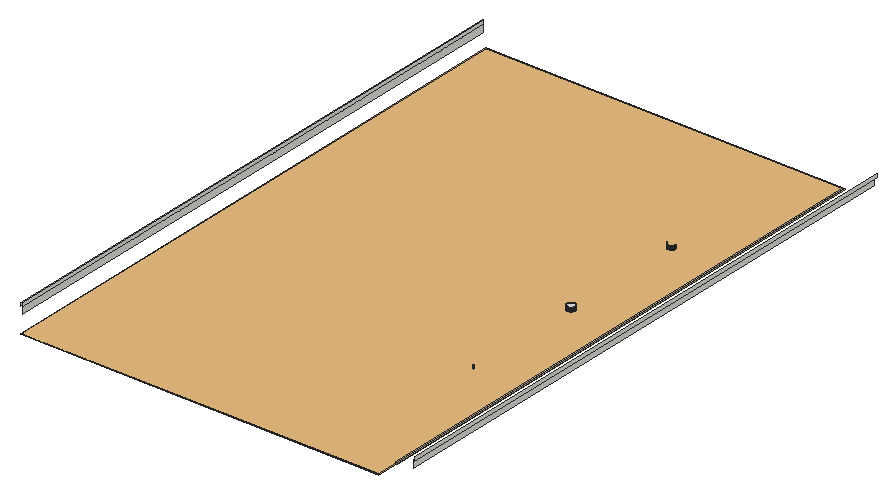
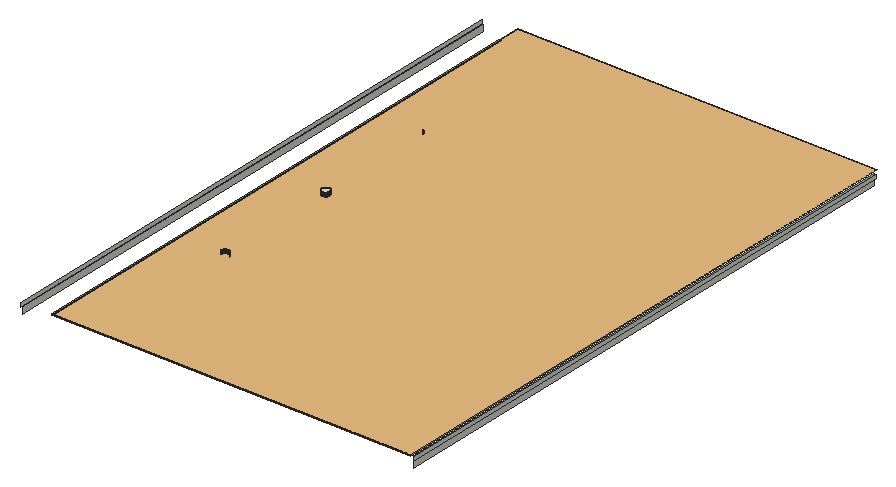
# SketchUp Ruby script. Lengths in inches.
U = 1.inch
M = Sketchup.active_model
def pt(a) = Geom::Point3d.new(a.map { |v| v * U })
def face(e, loops, mat)
  f = e.add_face(loops[0].map { |a| pt(a) })
  loops[1..].each { |l| e.add_face(l.map { |a| pt(a) }).erase! }
  f.material = f.back_material = mat if mat
  f
end
# faces: each face lists its corners as indices into pts; further lists are holes
def faces(e, pts, list, mat = nil) = list.each { |f| face(e, (f[0].is_a?(Array) ? f : [f]).map { |l| l.map { |i| pts[i] } }, mat) }
# xy, xz, yz: faces in a plane at the given z, y or x. An outline is a flat list of corners, or four numbers for a rectangle; further outlines are holes
def ring(l) = l.size == 4 ? [[l[0], l[1]], [l[2], l[1]], [l[2], l[3]], [l[0], l[3]]] : l.each_slice(2).to_a
def flat(e, list, mat, &to3) = list.each { |f| face(e, (f[0].is_a?(Array) ? f : [f]).map { |l| ring(l).map { |u, v| to3.(u, v) } }, mat) }
def xy(e, z, list, mat = nil) = flat(e, list, mat) { |x, y| [x, y, z] }
def xz(e, y, list, mat = nil) = flat(e, list, mat) { |x, z| [x, y, z] }
def yz(e, x, list, mat = nil) = flat(e, list, mat) { |y, z| [x, y, z] }
def lines(e, pts, list) = list.each { |a, b| e.add_line(pt(pts[a]), pt(pts[b])) }
# prism: a flat outline (further loops are holes) pulled along v
def prism(e, loops, v, mat = nil)
  f = face(e, loops, mat); d = Geom::Vector3d.new(v.map { |x| x * U })
  f.pushpull(f.normal.samedirection?(d) ? d.length : -d.length)
end
def box(e, o, s, mat = nil) = prism(e, [[o, [o[0] + s[0], o[1], o[2]], [o[0] + s[0], o[1] + s[1], o[2]], [o[0], o[1] + s[1], o[2]]]], [0, 0, s[2]], mat)
def at(x, y, z, deg = 0) = Geom::Transformation.translation(pt([x, y, z])) * Geom::Transformation.rotation(ORIGIN, Z_AXIS, deg.degrees)
def axes(o, x, y, z) = Geom::Transformation.new([*x, 0, *y, 0, *z, 0, *pt(o).to_a, 1])
def part(name) = M.definitions.add(name)
# library, detail: a bought-in or finely detailed component or shape, given as its bounding box
def library(name, o, s) = part(name).tap { |d| box(d.entities, o, s) }
def detail(e, o, s) = box(e.add_group.entities, o, s)
def put(e, d, t, mat = nil) = e.add_instance(d, t).tap { |i| i.material = mat if mat }
def group(e, t, mat = nil) = e.add_group.tap { |g| g.transformation = t; g.material = mat if mat }.entities
root = M.entities
M.materials.add("False ceiling Light").color = [253, 207, 127]
c1 = library("Group\#41",[0,0,-0.5],[265,430,0.5])
xy(root,351,[[251.84,435,251.76,435.01,251.6875,435.02,251.61,435.03,251.45,435.05,251.375,435.07,251.3,435.08,251.22,435.1,251.15,435.125,251.07,435.15,251,435.17,250.92,435.2,250.71,435.29,250.64,435.33,250.57,435.36,250.43,435.44,250.37,435.48,250.3,435.53,250.24,435.57,250.17,435.62,249.93,435.82,249.88,435.88,249.77,435.99,249.62,436.17,249.57,436.24,249.53,436.3,249.48,436.37,249.44,436.43,249.36,436.57,249.33,436.64,249.29,436.71,249.23,436.85,249.2,436.93,249.17,437,249.15,437.07,249.125,437.15,249.1,437.22,249.08,437.3,249.07,437.375,249.05,437.45,249.03,437.61,249.02,437.6875,249.01,437.76,249,437.84,249,438.16,249.01,438.24,249.02,438.3125,249.03,438.39,249.05,438.55,249.07,438.625,249.08,438.7,249.1,438.78,249.125,438.85,249.15,438.93,249.17,439,249.2,439.08,249.29,439.29,249.33,439.36,249.36,439.43,249.44,439.57,249.48,439.63,249.53,439.7,249.57,439.76,249.62,439.83,249.82,440.07,249.88,440.12,249.99,440.23,250.17,440.38,250.24,440.43,250.3,440.47,250.37,440.52,250.43,440.56,250.57,440.64,250.64,440.67,250.71,440.71,250.85,440.77,250.93,440.8,251,440.83,251.07,440.85,251.15,440.875,251.22,440.9,251.3,440.92,251.375,440.93,251.45,440.95,251.61,440.97,251.6875,440.98,251.76,440.99,251.84,441,252.16,441,252.24,440.99,252.3125,440.98,252.39,440.97,252.55,440.95,252.625,440.93,252.7,440.92,252.78,440.9,252.85,440.875,252.93,440.85,253,440.83,253.08,440.8,253.29,440.71,253.36,440.67,253.43,440.64,253.57,440.56,253.63,440.52,253.7,440.47,253.76,440.43,253.83,440.38,254.07,440.18,254.12,440.12,254.23,440.01,254.38,439.83,254.43,439.76,254.47,439.7,254.52,439.63,254.56,439.57,254.64,439.43,254.67,439.36,254.71,439.29,254.77,439.15,254.8,439.07,254.83,439,254.85,438.93,254.875,438.85,254.9,438.78,254.92,438.7,254.93,438.625,254.95,438.55,254.97,438.39,254.98,438.3125,254.99,438.24,255,438.16,255,437.84,254.99,437.76,254.98,437.6875,254.97,437.61,254.95,437.45,254.93,437.375,254.92,437.3,254.9,437.22,254.875,437.15,254.85,437.07,254.83,437,254.8,436.92,254.71,436.71,254.67,436.64,254.64,436.57,254.56,436.43,254.52,436.37,254.47,436.3,254.43,436.24,254.38,436.17,254.18,435.93,254.12,435.88,254.01,435.77,253.83,435.62,253.76,435.57,253.7,435.53,253.63,435.48,253.57,435.44,253.43,435.36,253.36,435.33,253.29,435.29,253.15,435.23,253.07,435.2,253,435.17,252.93,435.15,252.85,435.125,252.78,435.1,252.7,435.08,252.625,435.07,252.55,435.05,252.39,435.03,252.3125,435.02,252.24,435.01,252.16,435]])
xz(root,348,[[251.84,348,251.92,351],[251.92,348,252,351],[252,348,252.08,351],[252.08,348,252.16,351]])
xz(root,435,[[251.84,348,251.92,351],[251.92,348,252,351],[252,348,252.08,351],[252.08,348,252.16,351]])
xz(root,441,[[251.84,348,251.92,351],[251.92,348,252,351],[252,348,252.08,351],[252.08,348,252.16,351]])
xz(root,528,[[251.84,348,251.92,351],[251.92,348,252,351],[252,348,252.08,351],[252.08,348,252.16,351]])
yz(root,9,[[234,354.5,660,357]])
yz(root,10,[[234,349.5,659,354.5],[234,354.5,659,357]])
yz(root,249,[[437.84,348,437.92,351],[437.92,348,438,351],[438,348,438.08,351],[438.08,348,438.16,351]])
yz(root,255,[[437.84,348,437.92,351],[437.92,348,438,351],[438,348,438.08,351],[438.08,348,438.16,351]])
yz(root,286,[[234,348,646,348.5]])
yz(root,287,[[234,348,647,348.5]])
yz(root,299,[[234,349.5,659,354.5]])
yz(root,300,[[234,354.5,660,357]])
p = [[251.45,347.95,348],[251.53,347.96,348],[251.53,347.96,351],[251.45,347.95,351],[251.61,347.97,348],[251.61,347.97,351],
  [251.6875,347.98,348],[251.6875,347.98,351],[251.76,347.99,348],[251.76,347.99,351],[251.84,348,348],[251.84,348,351],
  [252.24,347.99,348],[252.3125,347.98,348],[252.3125,347.98,351],[252.24,347.99,351],[252.16,348,348],[252.16,348,351],
  [252.39,347.97,348],[252.39,347.97,351],[252.47,347.96,348],[252.47,347.96,351],[251.61,435.03,348],[251.53,435.04,348],
  [251.53,435.04,351],[251.61,435.03,351],[251.45,435.05,348],[251.45,435.05,351],[251.6875,435.02,348],[251.6875,435.02,351],
  [251.76,435.01,348],[251.76,435.01,351],[251.84,435,348],[251.84,435,351],[252.24,435.01,348],[252.16,435,348],
  [252.16,435,351],[252.24,435.01,351],[252.3125,435.02,348],[252.3125,435.02,351],[252.39,435.03,348],[252.39,435.03,351],
  [252.47,435.04,348],[252.47,435.04,351],[252.55,435.05,348],[252.55,435.05,351],[251.07,435.15,348],[251,435.17,348],
  [251,435.17,351],[251.07,435.15,351],[251.22,435.1,348],[251.15,435.125,348],[251.15,435.125,351],[251.22,435.1,351],
  [251.3,435.08,348],[251.3,435.08,351],[251.375,435.07,348],[251.375,435.07,351],[252.625,435.07,348],[252.625,435.07,351],
  [252.7,435.08,348],[252.7,435.08,351],[252.78,435.1,348],[252.78,435.1,351],[252.85,435.125,348],[252.85,435.125,351],
  [252.93,435.15,348],[252.93,435.15,351],[253,435.17,348],[253,435.17,351],[250.85,435.23,348],[250.78,435.26,348],
  [250.78,435.26,351],[250.85,435.23,351],[250.92,435.2,348],[250.92,435.2,351],[253.07,435.2,348],[253.07,435.2,351],
  [253.15,435.23,348],[253.15,435.23,351],[253.22,435.26,348],[253.22,435.26,351],[250.71,435.29,348],[250.64,435.33,348],
  [250.64,435.33,351],[250.71,435.29,351],[250.57,435.36,348],[250.57,435.36,351],[253.29,435.29,348],[253.29,435.29,351],
  [253.36,435.33,348],[253.36,435.33,351],[253.43,435.36,348],[253.43,435.36,351],[250.5,435.4,348],[250.43,435.44,348],
  [250.43,435.44,351],[250.5,435.4,351],[250.37,435.48,348],[250.37,435.48,351],[253.5,435.4,348],[253.5,435.4,351],
  [253.57,435.44,348],[253.57,435.44,351],[253.63,435.48,348],[253.63,435.48,351],[250.3,435.53,348],[250.24,435.57,348],
  [250.24,435.57,351],[250.3,435.53,351],[253.7,435.53,348],[253.7,435.53,351],[253.76,435.57,348],[253.76,435.57,351],
  [250.17,435.62,348],[250.11,435.67,348],[250.11,435.67,351],[250.17,435.62,351],[253.83,435.62,348],[253.83,435.62,351],
  [253.89,435.67,348],[253.89,435.67,351],[250.05,435.72,348],[249.99,435.77,348],[249.99,435.77,351],[250.05,435.72,351],
  [253.95,435.72,348],[253.95,435.72,351],[254.01,435.77,348],[254.01,435.77,351],[249.93,435.82,348],[249.93,435.82,351],
  [249.88,435.88,348],[249.88,435.88,351],[254.06,435.82,348],[254.06,435.82,351],[254.12,435.88,348],[254.12,435.88,351],
  [249.82,435.94,348],[249.82,435.94,351],[249.77,435.99,348],[249.77,435.99,351],[254.18,435.93,348],[254.18,435.93,351],
  [254.23,435.99,348],[254.23,435.99,351],[249.72,436.05,348],[249.72,436.05,351],[254.28,436.05,348],[254.28,436.05,351],
  [249.67,436.11,348],[249.62,436.17,348],[249.62,436.17,351],[249.67,436.11,351],[254.33,436.11,348],[254.33,436.11,351],
  [254.38,436.17,348],[254.38,436.17,351],[249.57,436.24,348],[249.53,436.3,348],[249.53,436.3,351],[249.57,436.24,351],
  [254.43,436.24,348],[254.43,436.24,351],[254.47,436.3,348],[254.47,436.3,351],[249.48,436.37,348],[249.48,436.37,351],
  [254.52,436.37,348],[254.52,436.37,351],[249.44,436.43,348],[249.44,436.43,351],[249.4,436.5,348],[249.4,436.5,351],
  [254.56,436.43,348],[254.56,436.43,351],[254.6,436.5,348],[254.6,436.5,351],[249.36,436.57,348],[249.36,436.57,351],
  [254.64,436.57,348],[254.64,436.57,351],[249.33,436.64,348],[249.33,436.64,351],[249.29,436.71,348],[249.29,436.71,351],
  [254.67,436.64,348],[254.67,436.64,351],[254.71,436.71,348],[254.71,436.71,351],[249.26,436.78,348],[249.26,436.78,351],
  [254.74,436.78,348],[254.74,436.78,351],[249.23,436.85,348],[249.23,436.85,351],[254.77,436.85,348],[254.77,436.85,351],
  [249.2,436.93,348],[249.2,436.93,351],[249.17,437,348],[249.17,437,351],[254.8,436.92,348],[254.8,436.92,351],
  [254.83,437,348],[254.83,437,351],[249.15,437.07,348],[249.15,437.07,351],[254.85,437.07,348],[254.85,437.07,351],
  [249.125,437.15,348],[249.125,437.15,351],[249.1,437.22,348],[249.1,437.22,351],[254.875,437.15,348],[254.875,437.15,351],
  [254.9,437.22,348],[254.9,437.22,351],[249.08,437.3,348],[249.08,437.3,351],[254.92,437.3,348],[254.92,437.3,351],
  [249.07,437.375,348],[249.07,437.375,351],[254.93,437.375,348],[254.93,437.375,351],[249.05,437.45,348],[249.05,437.45,351],
  [254.95,437.45,348],[254.95,437.45,351],[249.04,437.53,348],[249.04,437.53,351],[249.03,437.61,348],[249.03,437.61,351],
  [254.96,437.53,348],[254.96,437.53,351],[254.97,437.61,348],[254.97,437.61,351],[249.02,437.6875,348],[249.02,437.6875,351],
  [254.98,437.6875,348],[254.98,437.6875,351],[249.01,437.76,348],[249.01,437.76,351],[254.99,437.76,348],[254.99,437.76,351],
  [249,437.84,348],[249,437.84,351],[255,437.84,348],[255,437.84,351],[249,438.16,348],[249.01,438.24,348],
  [249.01,438.24,351],[249,438.16,351],[249.02,438.3125,348],[249.02,438.3125,351],[254.99,438.24,348],[255,438.16,348],
  [255,438.16,351],[254.99,438.24,351],[254.98,438.3125,348],[254.98,438.3125,351],[249.03,438.39,348],[249.03,438.39,351],
  [254.97,438.39,348],[254.97,438.39,351],[249.04,438.47,348],[249.04,438.47,351],[254.96,438.47,348],[254.96,438.47,351],
  [249.05,438.55,348],[249.05,438.55,351],[249.07,438.625,348],[249.07,438.625,351],[254.95,438.55,348],[254.95,438.55,351],
  [254.93,438.625,348],[254.93,438.625,351],[249.08,438.7,348],[249.08,438.7,351],[254.92,438.7,348],[254.92,438.7,351],
  [249.1,438.78,348],[249.1,438.78,351],[254.9,438.78,348],[254.9,438.78,351],[249.125,438.85,348],[249.125,438.85,351],
  [254.875,438.85,348],[254.875,438.85,351],[249.15,438.93,348],[249.15,438.93,351],[249.17,439,348],[249.17,439,351],
  [254.83,439,348],[254.85,438.93,348],[254.85,438.93,351],[254.83,439,351],[249.2,439.08,348],[249.2,439.08,351],
  [254.8,439.07,348],[254.8,439.07,351],[249.23,439.15,348],[249.23,439.15,351],[249.26,439.22,348],[249.26,439.22,351],
  [254.74,439.22,348],[254.77,439.15,348],[254.77,439.15,351],[254.74,439.22,351],[249.29,439.29,348],[249.29,439.29,351],
  [254.71,439.29,348],[254.71,439.29,351],[249.33,439.36,348],[249.33,439.36,351],[254.67,439.36,348],[254.67,439.36,351],
  [249.36,439.43,348],[249.36,439.43,351],[249.4,439.5,348],[249.4,439.5,351],[254.64,439.43,348],[254.64,439.43,351],
  [254.6,439.5,348],[254.6,439.5,351],[249.44,439.57,348],[249.44,439.57,351],[254.56,439.57,348],[254.56,439.57,351],
  [249.48,439.63,348],[249.48,439.63,351],[249.53,439.7,348],[249.53,439.7,351],[254.52,439.63,348],[254.52,439.63,351],
  [254.47,439.7,348],[254.47,439.7,351],[249.57,439.76,348],[249.57,439.76,351],[254.43,439.76,348],[254.43,439.76,351],
  [249.62,439.83,348],[249.62,439.83,351],[249.67,439.89,348],[249.67,439.89,351],[254.33,439.89,348],[254.38,439.83,348],
  [254.38,439.83,351],[254.33,439.89,351],[249.72,439.95,348],[249.72,439.95,351],[249.77,440.01,348],[249.77,440.01,351],
  [254.23,440.01,348],[254.28,439.95,348],[254.28,439.95,351],[254.23,440.01,351],[249.82,440.07,348],[249.82,440.07,351],
  [254.18,440.06,348],[254.18,440.06,351],[249.88,440.12,348],[249.88,440.12,351],[249.94,440.18,348],[249.94,440.18,351],
  [254.12,440.12,348],[254.12,440.12,351],[254.07,440.18,348],[254.07,440.18,351],[249.99,440.23,348],[249.99,440.23,351],
  [250.05,440.28,348],[250.05,440.28,351],[253.95,440.28,348],[254.01,440.23,348],[254.01,440.23,351],[253.95,440.28,351],
  [250.11,440.33,348],[250.11,440.33,351],[250.17,440.38,348],[250.17,440.38,351],[253.83,440.38,348],[253.89,440.33,348],
  [253.89,440.33,351],[253.83,440.38,351],[250.24,440.43,348],[250.24,440.43,351],[250.3,440.47,348],[250.3,440.47,351],
  [253.7,440.47,348],[253.76,440.43,348],[253.76,440.43,351],[253.7,440.47,351],[250.37,440.52,348],[250.37,440.52,351],
  [250.43,440.56,348],[250.43,440.56,351],[253.63,440.52,348],[253.63,440.52,351],[253.57,440.56,348],[253.57,440.56,351],
  [250.5,440.6,348],[250.5,440.6,351],[250.57,440.64,348],[250.57,440.64,351],[250.64,440.67,348],[250.64,440.67,351],
  [253.43,440.64,348],[253.5,440.6,348],[253.5,440.6,351],[253.43,440.64,351],[253.36,440.67,348],[253.36,440.67,351],
  [250.71,440.71,348],[250.71,440.71,351],[250.78,440.74,348],[250.78,440.74,351],[250.85,440.77,348],[250.85,440.77,351],
  [253.15,440.77,348],[253.22,440.74,348],[253.22,440.74,351],[253.15,440.77,351],[253.29,440.71,348],[253.29,440.71,351],
  [250.93,440.8,348],[250.93,440.8,351],[251,440.83,348],[251,440.83,351],[251.07,440.85,348],[251.07,440.85,351],
  [252.93,440.85,348],[253,440.83,348],[253,440.83,351],[252.93,440.85,351],[253.08,440.8,348],[253.08,440.8,351],
  [251.15,440.875,348],[251.15,440.875,351],[251.22,440.9,348],[251.22,440.9,351],[251.3,440.92,348],[251.3,440.92,351],
  [251.375,440.93,348],[251.375,440.93,351],[251.45,440.95,348],[251.45,440.95,351],[251.53,440.96,348],[251.53,440.96,351],
  [252.55,440.95,348],[252.625,440.93,348],[252.625,440.93,351],[252.55,440.95,351],[252.47,440.96,348],[252.47,440.96,351],
  [252.7,440.92,348],[252.7,440.92,351],[252.78,440.9,348],[252.78,440.9,351],[252.85,440.875,348],[252.85,440.875,351],
  [251.61,440.97,348],[251.61,440.97,351],[251.6875,440.98,348],[251.6875,440.98,351],[251.76,440.99,348],[251.76,440.99,351],
  [251.84,441,348],[251.84,441,351],[252.24,440.99,348],[252.3125,440.98,348],[252.3125,440.98,351],[252.24,440.99,351],
  [252.16,441,348],[252.16,441,351],[252.39,440.97,348],[252.39,440.97,351],[251.61,528.03,348],[251.53,528.04,348],
  [251.53,528.04,351],[251.61,528.03,351],[251.45,528.05,348],[251.45,528.05,351],[251.6875,528.02,348],[251.6875,528.02,351],
  [251.76,528.01,348],[251.76,528.01,351],[251.84,528,348],[251.84,528,351],[252.24,528.01,348],[252.16,528,348],
  [252.16,528,351],[252.24,528.01,351],[252.3125,528.02,348],[252.3125,528.02,351],[252.39,528.03,348],[252.39,528.03,351],
  [252.47,528.04,348],[252.47,528.04,351],[252.55,528.05,348],[252.55,528.05,351],[251.07,528.15,348],[251,528.17,348],
  [251,528.17,351],[251.07,528.15,351],[251.22,528.1,348],[251.15,528.125,348],[251.15,528.125,351],[251.22,528.1,351],
  [251.3,528.08,348],[251.3,528.08,351],[251.375,528.07,348],[251.375,528.07,351],[252.625,528.07,348],[252.625,528.07,351],
  [252.7,528.08,348],[252.7,528.08,351],[252.78,528.1,348],[252.78,528.1,351],[252.85,528.125,348],[252.85,528.125,351],
  [252.93,528.15,348],[252.93,528.15,351],[253,528.17,348],[253,528.17,351],[250.85,528.23,348],[250.78,528.26,348],
  [250.78,528.26,351],[250.85,528.23,351],[250.92,528.2,348],[250.92,528.2,351],[253.07,528.2,348],[253.07,528.2,351],
  [253.15,528.23,348],[253.15,528.23,351],[253.22,528.26,348],[253.22,528.26,351],[250.71,528.29,348],[250.64,528.33,348],
  [250.64,528.33,351],[250.71,528.29,351],[250.57,528.36,348],[250.57,528.36,351],[253.29,528.29,348],[253.29,528.29,351],
  [253.36,528.33,348],[253.36,528.33,351],[253.43,528.36,348],[253.43,528.36,351],[250.5,528.4,348],[250.43,528.44,348],
  [250.43,528.44,351],[250.5,528.4,351],[250.37,528.48,348],[250.37,528.48,351],[253.5,528.4,348],[253.5,528.4,351],
  [253.57,528.44,348],[253.57,528.44,351],[253.63,528.48,348],[253.63,528.48,351],[250.3,528.53,348],[250.24,528.57,348],
  [250.24,528.57,351],[250.3,528.53,351],[253.7,528.53,348],[253.7,528.53,351],[253.76,528.57,348],[253.76,528.57,351],
  [250.17,528.62,348],[250.11,528.67,348],[250.11,528.67,351],[250.17,528.62,351],[253.83,528.62,348],[253.83,528.62,351],
  [253.89,528.67,348],[253.89,528.67,351],[250.05,528.72,348],[249.99,528.77,348],[249.99,528.77,351],[250.05,528.72,351],
  [253.95,528.72,348],[253.95,528.72,351],[254.01,528.77,348],[254.01,528.77,351],[249.93,528.82,348],[249.93,528.82,351],
  [249.88,528.88,348],[249.88,528.88,351],[254.06,528.82,348],[254.06,528.82,351],[254.12,528.88,348],[254.12,528.88,351],
  [249.82,528.94,348],[249.82,528.94,351],[249.77,528.99,348],[249.77,528.99,351],[254.18,528.93,348],[254.18,528.93,351],
  [254.23,528.99,348],[254.23,528.99,351],[249.72,529.05,348],[249.72,529.05,351],[254.28,529.05,348],[254.28,529.05,351],
  [249.67,529.11,348],[249.62,529.17,348],[249.62,529.17,351],[249.67,529.11,351],[254.33,529.11,348],[254.33,529.11,351],
  [254.38,529.17,348],[254.38,529.17,351],[249.57,529.24,348],[249.53,529.3,348],[249.53,529.3,351],[249.57,529.24,351],
  [254.43,529.24,348],[254.43,529.24,351],[254.47,529.3,348],[254.47,529.3,351],[249.48,529.37,348],[249.48,529.37,351],
  [254.52,529.37,348],[254.52,529.37,351],[249.44,529.43,348],[249.44,529.43,351],[249.4,529.5,348],[249.4,529.5,351],
  [254.56,529.43,348],[254.56,529.43,351],[254.6,529.5,348],[254.6,529.5,351],[249.36,529.57,348],[249.36,529.57,351],
  [254.64,529.57,348],[254.64,529.57,351],[249.33,529.64,348],[249.33,529.64,351],[249.29,529.71,348],[249.29,529.71,351],
  [254.67,529.64,348],[254.67,529.64,351],[254.71,529.71,348],[254.71,529.71,351],[249.26,529.78,348],[249.26,529.78,351],
  [254.74,529.78,348],[254.74,529.78,351],[249.23,529.85,348],[249.23,529.85,351],[254.77,529.85,348],[254.77,529.85,351],
  [249.2,529.93,348],[249.2,529.93,351],[249.17,530,348],[249.17,530,351],[254.8,529.92,348],[254.8,529.92,351],
  [254.83,530,348],[254.83,530,351],[249.15,530.07,348],[249.15,530.07,351],[254.85,530.07,348],[254.85,530.07,351],
  [249.125,530.15,348],[249.125,530.15,351],[249.1,530.22,348],[249.1,530.22,351],[254.875,530.15,348],[254.875,530.15,351],
  [254.9,530.22,348],[254.9,530.22,351],[249.08,530.3,348],[249.08,530.3,351],[254.92,530.3,348],[254.92,530.3,351],
  [249.07,530.375,348],[249.07,530.375,351],[254.93,530.375,348],[254.93,530.375,351],[249.05,530.45,348],[249.05,530.45,351],
  [254.95,530.45,348],[254.95,530.45,351],[249.04,530.53,348],[249.04,530.53,351],[249.03,530.61,348],[249.03,530.61,351],
  [254.96,530.53,348],[254.96,530.53,351],[254.97,530.61,348],[254.97,530.61,351],[249.02,530.6875,348],[249.02,530.6875,351],
  [254.98,530.6875,348],[254.98,530.6875,351],[254.99,530.76,348],[254.99,530.76,351]]
faces(root,p,[[0,1,2,3],[1,4,5,2],[4,6,7,5],[6,8,9,7],[8,10,11,9],[12,13,14,15],[16,12,15,17],[13,18,19,14],
  [18,20,21,19],[22,23,24,25],[23,26,27,24],[28,22,25,29],[30,28,29,31],[32,30,31,33],[34,35,36,37],[38,34,37,39],
  [40,38,39,41],[42,40,41,43],[44,42,43,45],[46,47,48,49],[50,51,52,53],[51,46,49,52],[54,50,53,55],[56,54,55,57],
  [26,56,57,27],[58,44,45,59],[60,58,59,61],[62,60,61,63],[64,62,63,65],[66,64,65,67],[68,66,67,69],[70,71,72,73],
  [47,74,75,48],[74,70,73,75],[76,68,69,77],[78,76,77,79],[80,78,79,81],[82,83,84,85],[83,86,87,84],[71,82,85,72],
  [88,80,81,89],[90,88,89,91],[92,90,91,93],[94,95,96,97],[95,98,99,96],[86,94,97,87],[100,92,93,101],[102,100,101,103],
  [104,102,103,105],[106,107,108,109],[98,106,109,99],[110,104,105,111],[112,110,111,113],[114,115,116,117],[107,114,117,108],[118,112,113,119],
  [120,118,119,121],[122,123,124,125],[115,122,125,116],[126,120,121,127],[128,126,127,129],[123,130,131,124],[130,132,133,131],[134,128,129,135],
  [136,134,135,137],[132,138,139,133],[138,140,141,139],[142,136,137,143],[144,142,143,145],[140,146,147,141],[148,144,145,149],[150,151,152,153],
  [146,150,153,147],[154,148,149,155],[156,154,155,157],[158,159,160,161],[151,158,161,152],[162,156,157,163],[164,162,163,165],[159,166,167,160],
  [168,164,165,169],[166,170,171,167],[170,172,173,171],[174,168,169,175],[176,174,175,177],[172,178,179,173],[180,176,177,181],[178,182,183,179],
  [182,184,185,183],[186,180,181,187],[188,186,187,189],[184,190,191,185],[192,188,189,193],[190,194,195,191],[196,192,193,197],[194,198,199,195],
  [198,200,201,199],[202,196,197,203],[204,202,203,205],[200,206,207,201],[208,204,205,209],[206,210,211,207],[210,212,213,211],[214,208,209,215],
  [216,214,215,217],[212,218,219,213],[220,216,217,221],[218,222,223,219],[224,220,221,225],[222,226,227,223],[228,224,225,229],[226,230,231,227],
  [230,232,233,231],[234,228,229,235],[236,234,235,237],[232,238,239,233],[240,236,237,241],[238,242,243,239],[244,240,241,245],[242,246,247,243],
  [248,244,245,249],[250,251,252,253],[251,254,255,252],[256,257,258,259],[260,256,259,261],[254,262,263,255],[264,260,261,265],[262,266,267,263],
  [268,264,265,269],[266,270,271,267],[270,272,273,271],[274,268,269,275],[276,274,275,277],[272,278,279,273],[280,276,277,281],[278,282,283,279],
  [284,280,281,285],[282,286,287,283],[288,284,285,289],[286,290,291,287],[290,292,293,291],[294,295,296,297],[295,288,289,296],[292,298,299,293],
  [300,294,297,301],[298,302,303,299],[302,304,305,303],[306,307,308,309],[307,300,301,308],[304,310,311,305],[312,306,309,313],[310,314,315,311],
  [316,312,313,317],[314,318,319,315],[318,320,321,319],[322,316,317,323],[324,322,323,325],[320,326,327,321],[328,324,325,329],[326,330,331,327],
  [330,332,333,331],[334,328,329,335],[336,334,335,337],[332,338,339,333],[340,336,337,341],[338,342,343,339],[342,344,345,343],[346,347,348,349],
  [347,340,341,348],[344,350,351,345],[350,352,353,351],[354,355,356,357],[355,346,349,356],[352,358,359,353],[360,354,357,361],[358,362,363,359],
  [362,364,365,363],[366,360,361,367],[368,366,367,369],[364,370,371,365],[370,372,373,371],[374,375,376,377],[375,368,369,376],[372,378,379,373],
  [378,380,381,379],[382,383,384,385],[383,374,377,384],[380,386,387,381],[386,388,389,387],[390,391,392,393],[391,382,385,392],[388,394,395,389],
  [394,396,397,395],[398,390,393,399],[400,398,399,401],[396,402,403,397],[402,404,405,403],[404,406,407,405],[408,409,410,411],[412,408,411,413],
  [409,400,401,410],[406,414,415,407],[414,416,417,415],[416,418,419,417],[420,421,422,423],[421,424,425,422],[424,412,413,425],[418,426,427,419],
  [426,428,429,427],[428,430,431,429],[432,433,434,435],[433,436,437,434],[436,420,423,437],[430,438,439,431],[438,440,441,439],[440,442,443,441],
  [442,444,445,443],[444,446,447,445],[446,448,449,447],[450,451,452,453],[454,450,453,455],[451,456,457,452],[456,458,459,457],[458,460,461,459],
  [460,432,435,461],[448,462,463,449],[462,464,465,463],[464,466,467,465],[466,468,469,467],[470,471,472,473],[474,470,473,475],[471,476,477,472],
  [476,454,455,477],[478,479,480,481],[479,482,483,480],[484,478,481,485],[486,484,485,487],[488,486,487,489],[490,491,492,493],[494,490,493,495],
  [496,494,495,497],[498,496,497,499],[500,498,499,501],[502,503,504,505],[506,507,508,509],[507,502,505,508],[510,506,509,511],[512,510,511,513],
  [482,512,513,483],[514,500,501,515],[516,514,515,517],[518,516,517,519],[520,518,519,521],[522,520,521,523],[524,522,523,525],[526,527,528,529],
  [503,530,531,504],[530,526,529,531],[532,524,525,533],[534,532,533,535],[536,534,535,537],[538,539,540,541],[539,542,543,540],[527,538,541,528],
  [544,536,537,545],[546,544,545,547],[548,546,547,549],[550,551,552,553],[551,554,555,552],[542,550,553,543],[556,548,549,557],[558,556,557,559],
  [560,558,559,561],[562,563,564,565],[554,562,565,555],[566,560,561,567],[568,566,567,569],[570,571,572,573],[563,570,573,564],[574,568,569,575],
  [576,574,575,577],[578,579,580,581],[571,578,581,572],[582,576,577,583],[584,582,583,585],[579,586,587,580],[586,588,589,587],[590,584,585,591],
  [592,590,591,593],[588,594,595,589],[594,596,597,595],[598,592,593,599],[600,598,599,601],[596,602,603,597],[604,600,601,605],[606,607,608,609],
  [602,606,609,603],[610,604,605,611],[612,610,611,613],[614,615,616,617],[607,614,617,608],[618,612,613,619],[620,618,619,621],[615,622,623,616],
  [624,620,621,625],[622,626,627,623],[626,628,629,627],[630,624,625,631],[632,630,631,633],[628,634,635,629],[636,632,633,637],[634,638,639,635],
  [638,640,641,639],[642,636,637,643],[644,642,643,645],[640,646,647,641],[648,644,645,649],[646,650,651,647],[652,648,649,653],[650,654,655,651],
  [654,656,657,655],[658,652,653,659],[660,658,659,661],[656,662,663,657],[664,660,661,665],[662,666,667,663],[666,668,669,667],[670,664,665,671],
  [672,670,671,673],[668,674,675,669],[676,672,673,677],[674,678,679,675],[680,676,677,681],[678,682,683,679],[684,680,681,685],[682,686,687,683],
  [686,688,689,687],[690,684,685,691],[692,690,691,693],[688,694,695,689],[696,692,693,697],[698,696,697,699]])
put(root,c1,at(22,217,348.5),"False ceiling Light")
